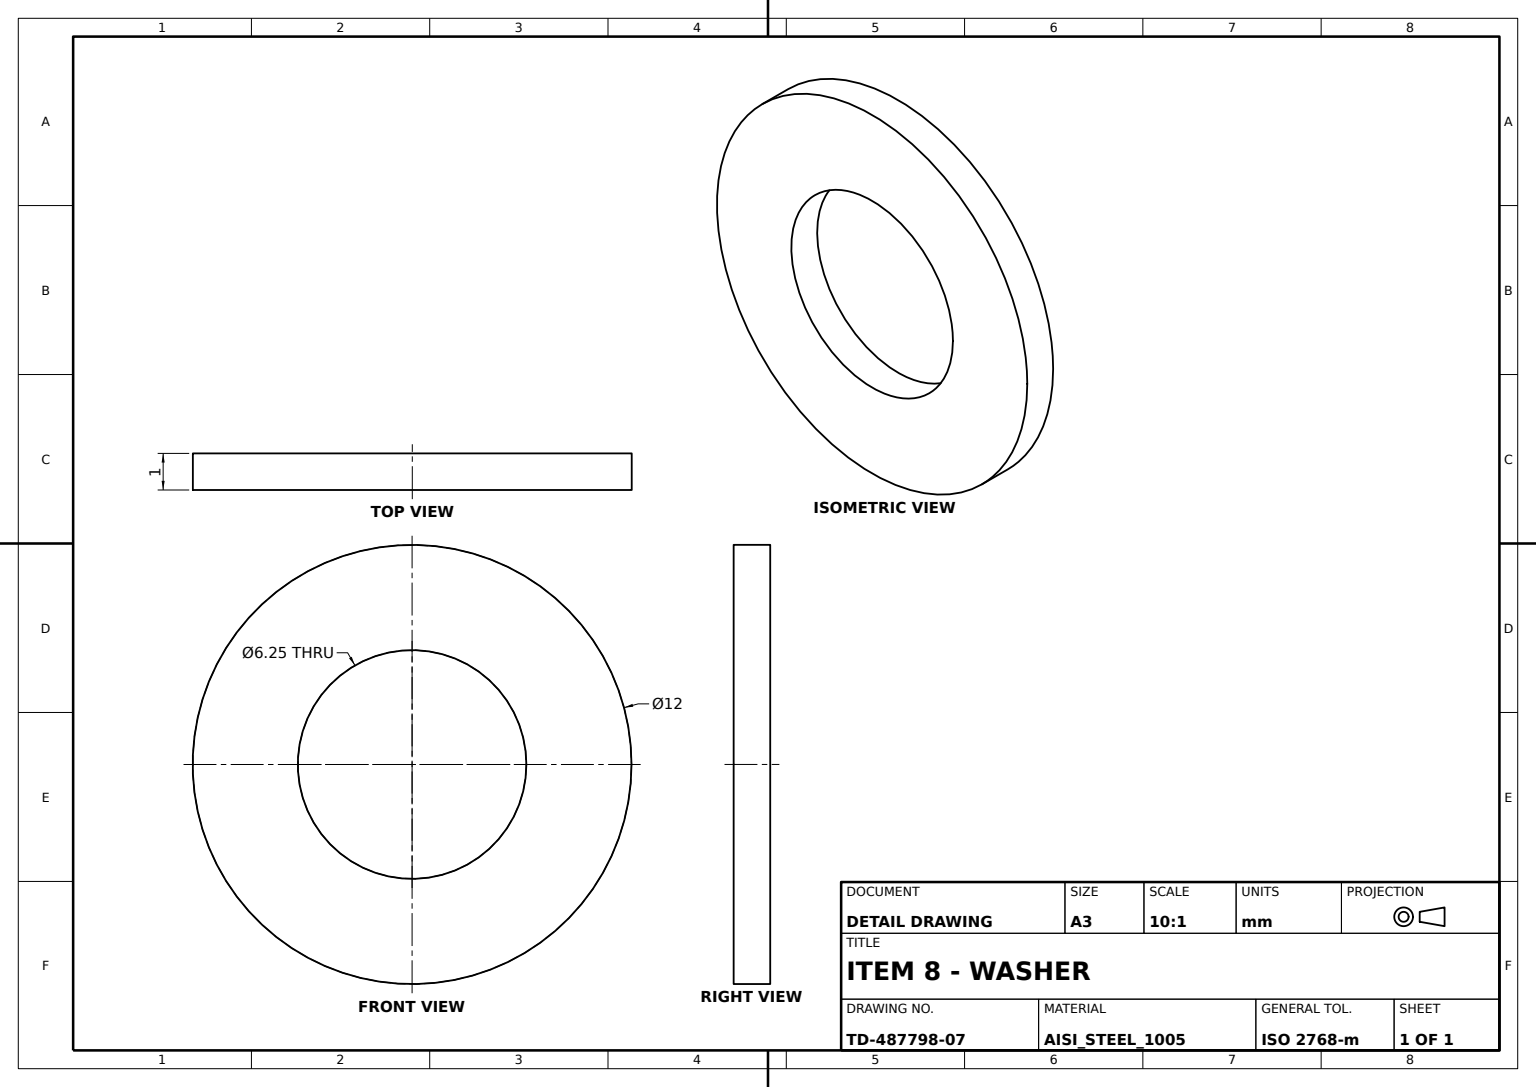
ISO-10303-21;
HEADER;
FILE_DESCRIPTION((''),'2;1');
FILE_NAME('','',(''),(''),'','','');
FILE_SCHEMA(('AUTOMOTIVE_DESIGN'));
ENDSEC;
DATA;
#1=APPLICATION_CONTEXT('');
#2=PRODUCT_CONTEXT('',#1,'mechanical');
#3=PRODUCT('','','',(#2));
#4=PRODUCT_DEFINITION_FORMATION('','',#3);
#5=PRODUCT_DEFINITION_CONTEXT('',#1,'design');
#6=PRODUCT_DEFINITION('','',#4,#5);
#7=PRODUCT_DEFINITION_SHAPE('','',#6);
#8=(LENGTH_UNIT()NAMED_UNIT(*)SI_UNIT(.MILLI.,.METRE.));
#9=(NAMED_UNIT(*)PLANE_ANGLE_UNIT()SI_UNIT($,.RADIAN.));
#10=(NAMED_UNIT(*)SI_UNIT($,.STERADIAN.)SOLID_ANGLE_UNIT());
#11=UNCERTAINTY_MEASURE_WITH_UNIT(LENGTH_MEASURE(0.005),#8,'distance_accuracy_value','');
#12=(GEOMETRIC_REPRESENTATION_CONTEXT(3)GLOBAL_UNCERTAINTY_ASSIGNED_CONTEXT((#11))GLOBAL_UNIT_ASSIGNED_CONTEXT((#8,#9,#10))REPRESENTATION_CONTEXT('',''));
#13=CARTESIAN_POINT('',(3.125,0.,0.));
#14=VERTEX_POINT('',#13);
#15=CARTESIAN_POINT('',(0.,0.,0.));
#16=DIRECTION('',(0.,0.,-1.));
#17=DIRECTION('',(1.,0.,0.));
#18=AXIS2_PLACEMENT_3D('',#15,#16,#17);
#19=CIRCLE('',#18,3.125);
#20=EDGE_CURVE('',#14,#14,#19,.T.);
#21=ORIENTED_EDGE('',*,*,#20,.F.);
#22=EDGE_LOOP('',(#21));
#23=FACE_BOUND('',#22,.T.);
#24=CARTESIAN_POINT('',(6.,0.,0.));
#25=VERTEX_POINT('',#24);
#26=CIRCLE('',#18,6.);
#27=EDGE_CURVE('',#25,#25,#26,.T.);
#28=ORIENTED_EDGE('',*,*,#27,.T.);
#29=EDGE_LOOP('',(#28));
#30=FACE_BOUND('',#29,.T.);
#31=DIRECTION('',(-1.,0.,0.));
#32=AXIS2_PLACEMENT_3D('',#15,#16,#31);
#33=PLANE('',#32);
#34=ADVANCED_FACE('',(#23,#30),#33,.T.);
#35=ORIENTED_EDGE('',*,*,#20,.T.);
#36=EDGE_LOOP('',(#35));
#37=FACE_BOUND('',#36,.T.);
#38=CARTESIAN_POINT('',(3.125,0.,1.));
#39=VERTEX_POINT('',#38);
#40=CARTESIAN_POINT('',(0.,0.,1.));
#41=AXIS2_PLACEMENT_3D('',#40,#16,#17);
#42=CIRCLE('',#41,3.125);
#43=EDGE_CURVE('',#39,#39,#42,.T.);
#44=ORIENTED_EDGE('',*,*,#43,.F.);
#45=EDGE_LOOP('',(#44));
#46=FACE_BOUND('',#45,.T.);
#47=AXIS2_PLACEMENT_3D('',#40,#16,#31);
#48=CYLINDRICAL_SURFACE('',#47,3.125);
#49=ADVANCED_FACE('',(#37,#46),#48,.F.);
#50=CARTESIAN_POINT('',(6.,0.,1.));
#51=VERTEX_POINT('',#50);
#52=CIRCLE('',#41,6.);
#53=EDGE_CURVE('',#51,#51,#52,.T.);
#54=ORIENTED_EDGE('',*,*,#53,.T.);
#55=EDGE_LOOP('',(#54));
#56=FACE_BOUND('',#55,.T.);
#57=ORIENTED_EDGE('',*,*,#27,.F.);
#58=EDGE_LOOP('',(#57));
#59=FACE_BOUND('',#58,.T.);
#60=CYLINDRICAL_SURFACE('',#47,6.);
#61=ADVANCED_FACE('',(#56,#59),#60,.T.);
#62=ORIENTED_EDGE('',*,*,#53,.F.);
#63=EDGE_LOOP('',(#62));
#64=FACE_BOUND('',#63,.T.);
#65=ORIENTED_EDGE('',*,*,#43,.T.);
#66=EDGE_LOOP('',(#65));
#67=FACE_BOUND('',#66,.T.);
#68=PLANE('',#47);
#69=ADVANCED_FACE('',(#64,#67),#68,.F.);
#70=CLOSED_SHELL('',(#34,#49,#61,#69));
#71=MANIFOLD_SOLID_BREP('',#70);
#72=ADVANCED_BREP_SHAPE_REPRESENTATION('',(#71),#12);
#73=SHAPE_DEFINITION_REPRESENTATION(#7,#72);
ENDSEC;
END-ISO-10303-21;
